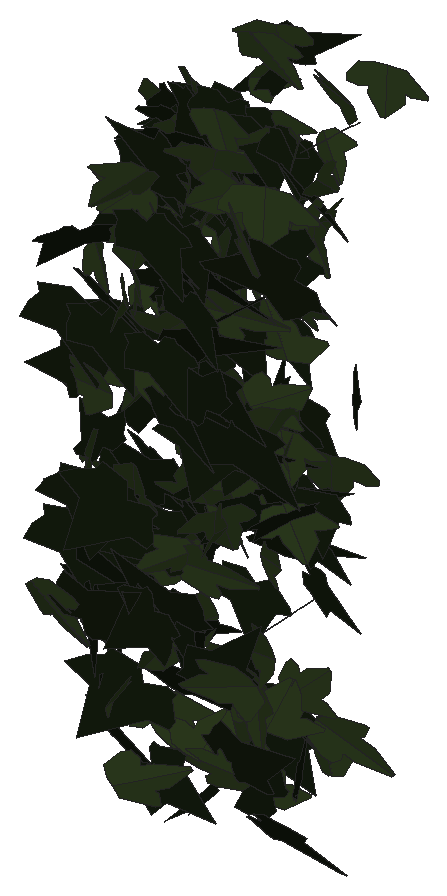
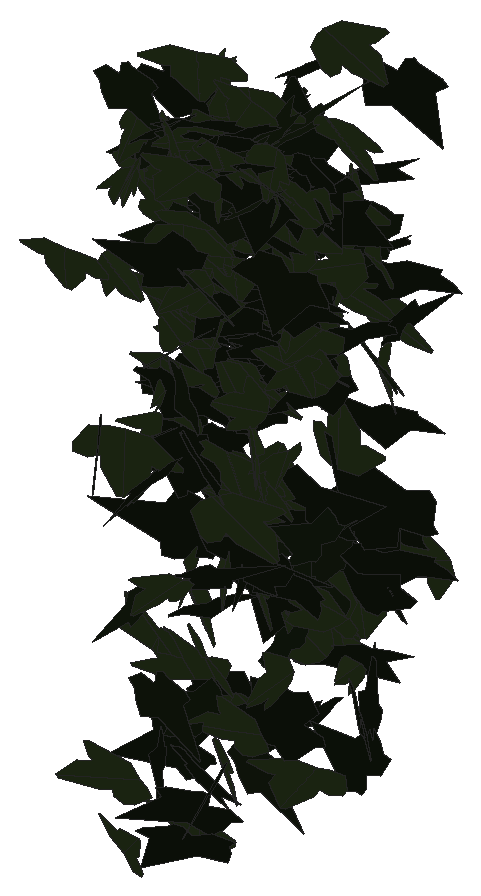
# SketchUp Ruby script. Lengths in millimetres.
U = 1.mm
M = Sketchup.active_model
def pt(a) = Geom::Point3d.new(a.map { |v| v * U })
def face(e, loops, mat)
  f = e.add_face(loops[0].map { |a| pt(a) })
  loops[1..].each { |l| e.add_face(l.map { |a| pt(a) }).erase! }
  f.material = f.back_material = mat if mat
  f
end
# faces: each face lists its corners as indices into pts; further lists are holes
def faces(e, pts, list, mat = nil) = list.each { |f| face(e, (f[0].is_a?(Array) ? f : [f]).map { |l| l.map { |i| pts[i] } }, mat) }
# xy, xz, yz: faces in a plane at the given z, y or x. An outline is a flat list of corners, or four numbers for a rectangle; further outlines are holes
def ring(l) = l.size == 4 ? [[l[0], l[1]], [l[2], l[1]], [l[2], l[3]], [l[0], l[3]]] : l.each_slice(2).to_a
def flat(e, list, mat, &to3) = list.each { |f| face(e, (f[0].is_a?(Array) ? f : [f]).map { |l| ring(l).map { |u, v| to3.(u, v) } }, mat) }
def xy(e, z, list, mat = nil) = flat(e, list, mat) { |x, y| [x, y, z] }
def xz(e, y, list, mat = nil) = flat(e, list, mat) { |x, z| [x, y, z] }
def yz(e, x, list, mat = nil) = flat(e, list, mat) { |y, z| [x, y, z] }
def lines(e, pts, list) = list.each { |a, b| e.add_line(pt(pts[a]), pt(pts[b])) }
# prism: a flat outline (further loops are holes) pulled along v
def prism(e, loops, v, mat = nil)
  f = face(e, loops, mat); d = Geom::Vector3d.new(v.map { |x| x * U })
  f.pushpull(f.normal.samedirection?(d) ? d.length : -d.length)
end
def box(e, o, s, mat = nil) = prism(e, [[o, [o[0] + s[0], o[1], o[2]], [o[0] + s[0], o[1] + s[1], o[2]], [o[0], o[1] + s[1], o[2]]]], [0, 0, s[2]], mat)
def at(x, y, z, deg = 0) = Geom::Transformation.translation(pt([x, y, z])) * Geom::Transformation.rotation(ORIGIN, Z_AXIS, deg.degrees)
def axes(o, x, y, z) = Geom::Transformation.new([*x, 0, *y, 0, *z, 0, *pt(o).to_a, 1])
def part(name) = M.definitions.add(name)
# library, detail: a bought-in or finely detailed component or shape, given as its bounding box
def library(name, o, s) = part(name).tap { |d| box(d.entities, o, s) }
def detail(e, o, s) = box(e.add_group.entities, o, s)
def put(e, d, t, mat = nil) = e.add_instance(d, t).tap { |i| i.material = mat if mat }
def group(e, t, mat = nil) = e.add_group.tap { |g| g.transformation = t; g.material = mat if mat }.entities
root = M.entities
M.materials.add("efeu1").color = [18, 25, 13]
M.materials.add("efeu2").color = [43, 57, 29]
c1 = part("ivyleaf_10")
p = [[0,12.8,-0.8],[-1.5,51.3,-10.9],[-4.9,51,-11.6],[-13.6,26.5,-7.3],[-13.2,15.9,-4.6],[-21.1,19.3,-7.2],
  [-29.5,16.3,-8.3],[-29.2,8.3,-6.2],[-19.7,-9.8,0.5],[-7.6,-13,4],[1,-12.2,5.8],[-0.4,51.1,-11.1],
  [-1.5,51.1,-10.9],[1,-12.4,5.9],[16.9,-12.4,3.5],[35.1,9.1,-5.1],[35,12.9,-6.1],[20.5,16.4,-4.9],
  [15.8,15,-3.8],[15.3,27.6,-7.1],[12.8,31.3,-7.8]]
faces(c1.entities,p,[[0,1,2,3,4,5,6,7,8,9,10],[11,12,0,13,14,15,16,17,18,19,20]],"efeu2")
c2 = part("ivyleaf_9")
p = [[39.1,54.8,31.7],[34.5,51.8,30.2],[-5.3,25.2,17.3],[-17.9,28.3,20.9],[-21.6,21.7,17],[-20.2,4.3,5.3],
  [-22.9,-0.3,2.5],[-17.1,-4,-0.6],[-2,-2.1,-1.2],[-0.7,-15.4,-10.1],[16.6,-22.3,-16.7],[21.1,-15.1,-12.5],
  [32.7,-10.7,-11],[46.1,-1.8,-6.6],[30.8,11.2,3.8]]
faces(c2.entities,p,[[0,1,2,3,4,5,6,7,8,9,10,11,12,13,14]],"efeu1")
put(root,c1,axes([4556.2,886.3,2542.8],[-1.01789,-0.02065,0.83927],[1.59777,-0.01294,0.53467],[-0.00035,0.99511,0.02437]))
put(root,c1,axes([4564.5,800.2,2431.5],[-0.15925,-0.13791,-1.07502],[1.36835,0.79977,-0.15856],[1.54355,-0.72322,0.02966]))
put(root,c2,axes([4578,723.1,2008.1],[-1.48385,-0.90702,-0.51552],[0.68416,0.37061,-1.19572],[1.86399,-0.85807,0.02849]))
put(root,c2,axes([4589.1,884.2,2448.3],[1.00623,0.8494,0.01435],[-0.12424,0.05747,-0.99682],[-1.61203,0.52577,0.08578]))
put(root,c1,axes([4580.1,1062.6,2511.9],[0.29812,0.25276,0.98298],[0.01179,0.99436,-0.25667],[-1.93162,0.04508,0.15014]))
put(root,c1,axes([4590.7,898.3,1915.5],[0.05878,0.11792,1.18277],[-0.48253,1.15659,-0.10869],[-2.21014,-0.24938,0.05519]))
put(root,c2,axes([4562.9,879.8,2561.1],[-0.31901,-0.00421,-0.99195],[1.88694,-0.03292,-0.16739],[-0.06044,-1.00548,0.00963]))
put(root,c1,axes([4594.7,1074.8,2581.2],[-1.55595,-0.56385,-0.01805],[0.12923,-0.0668,-0.98872],[1.06587,-0.81501,0.09352]))
put(root,c2,axes([4602.9,672.6,2277.1],[-0.44868,-0.18916,1.08119],[-1.24522,-0.86368,-0.29377],[1.67727,-0.69181,0.07113]))
put(root,c2,axes([4588.7,882.6,2406.1],[-1.19193,-0.69699,-0.34339],[0.4298,0.25873,-0.93701],[1.41492,-0.66573,-0.00464]))
put(root,c2,axes([4615.5,1063,2540],[-1.43483,0.68328,-0.16283],[0.23834,-0.10429,-1.01745],[-1.31542,-0.76421,-0.00674]))
put(root,c2,axes([4603.7,784.6,2473.6],[-0.07835,0.14297,-1.10614],[0.505,-1.07385,-0.14867],[-2.06176,-0.26846,0.00562]))
put(root,c1,axes([4571,734.4,2406.6],[0.64735,-0.2863,0.97578],[1.41515,-0.63187,-0.44459],[1.32025,0.81767,-0.00191]))
put(root,c2,axes([4577.1,786.8,2077.3],[0.3731,-1.04949,-0.00303],[0.00253,0.00333,-1.06764],[1.9974,0.19603,0.00192]))
put(root,c1,axes([4607.4,861.8,2487.1],[-1.5951,-0.65835,0.06001],[-0.07709,-0.04559,-1.06571],[1.2558,-0.83902,0.01081]))
put(root,c1,axes([4600.5,857.5,2305.2],[0.63665,0.81783,-0.44955],[-0.45449,-0.38665,-0.88109],[-1.71702,0.40559,0.06653]))
put(root,c2,axes([4586.6,758.1,1813],[-0.75692,0.17693,-1.07008],[1.82045,-0.4801,-0.43488],[-0.97314,-1.03574,0.01878]))
put(root,c2,axes([4617.2,822.9,2549.4],[0.46753,0.88942,-0.62998],[-0.37153,-0.59944,-0.92242],[-2.04081,0.31289,0.0236]))
put(root,c2,axes([4565.5,715.1,2049.6],[2.44799,0.26152,-0.16077],[0.2964,0.0409,1.31254],[0.50348,-1.29561,0.00898]))
put(root,c1,axes([4619.6,842.2,2526.7],[-1.77865,-0.22475,0.28094],[-0.52628,-0.05155,-0.9611],[0.43804,-0.97451,-0.01395]))
put(root,c2,axes([4596.3,724.5,1777.2],[0.27027,0.38621,1.16865],[-0.748,-1.10058,0.41147],[2.21984,-0.41788,-0.00364]))
put(root,c1,axes([4578.7,627.4,1960.3],[-1.14106,0.4755,-0.89578],[1.30933,-0.57389,-0.76508],[-1.41816,-0.91244,0.01439]))
put(root,c1,axes([4615.8,884,2593.4],[-1.44399,0.61214,0.2255],[-0.38212,0.10997,-0.97407],[-1.1813,-0.78384,0.03944]))
put(root,c2,axes([4581.2,837.7,2072.2],[0.73389,-0.86651,0.45505],[0.40083,-0.40417,-0.9481],[1.81907,0.43864,0.02533]))
put(root,c1,axes([4592.2,1047,2575.4],[-1.53117,0.15219,-0.61559],[1.07106,-0.28695,-0.80643],[-0.5562,-0.97153,0.14175]))
put(root,c2,axes([4592.3,802.4,2529.4],[0.55445,-0.97442,-0.31232],[-0.14144,0.30373,-1.01693],[1.94231,0.30027,0.0151]))
put(root,c2,axes([4600.4,754.5,2313.2],[-0.35988,-1.0455,-0.36243],[0.06215,0.36225,-1.06202],[2.10505,-0.18943,-0.03061]))
put(root,c2,axes([4647.8,774.1,2070],[0.13444,-0.08019,1.08996],[-1.54625,0.72671,0.10612],[-1.39127,-0.81541,-0.01261]))
put(root,c1,axes([4648.1,643,2274.6],[0.41932,-0.17233,-1.04982],[-1.60413,0.6259,-0.27963],[1.23547,0.87115,-0.00676]))
put(root,c2,axes([4587.8,1090.2,2547.4],[0.2442,0.07802,0.98269],[1.79038,0.28649,-0.14558],[-0.56074,0.94872,-0.03686]))
put(root,c2,axes([4646.6,884.6,2562.2],[-1.69221,0.45497,0.07745],[-0.31001,-0.15206,-0.97668],[-0.82184,-0.87946,0.20894]))
put(root,c2,axes([4607.4,676.5,2362.5],[-1.42898,-0.89142,-0.58993],[0.73571,0.44569,-1.16547],[1.89672,-0.84446,0.00762]))
put(root,c2,axes([4628.6,712.7,1939.7],[1.62408,-0.41988,0.80531],[-1.33457,0.39762,0.95037],[-1.09844,-1.10391,0.03601]))
put(root,c1,axes([4615.6,840.9,2560.2],[-0.80724,-0.71462,-0.56248],[0.56916,0.47653,-0.83094],[1.63458,-0.51885,0.01155]))
put(root,c2,axes([4602.5,681.1,1919.7],[-0.31423,0.70017,0.81678],[0.36351,-0.79414,0.71937],[2.01496,0.25246,-0.0024]))
put(root,c1,axes([4607.4,890.4,2541.2],[-0.35672,0.4667,-0.86016],[0.43813,-0.83019,-0.5006],[-1.81023,-0.2929,0.04834]))
put(root,c2,axes([4633.9,842,2564.4],[1.42432,0.43766,-0.76082],[-1.30135,-0.33618,-0.86598],[-1.04738,1.01287,0.04132]))
put(root,c2,axes([4626.8,881.9,2547.5],[1.37489,0.60815,-0.343],[-0.57756,-0.17102,-0.94235],[-1.19676,0.7812,0.06073]))
put(root,c2,axes([4591,742,1722.2],[0.56627,-0.59523,0.94998],[0.72797,-0.86999,-0.66491],[2.00556,0.48385,-0.02689]))
put(root,c1,axes([4605.5,773.7,2357.6],[-0.3705,0.12924,1.16872],[1.41357,-0.90487,0.22378],[1.7349,0.76487,0.06726]))
put(root,c1,axes([4621.5,853.6,2181.5],[0.37836,1.03837,-0.09617],[-0.03412,-0.09448,-1.05723],[-1.98439,0.19961,-0.00016]))
put(root,c2,axes([4654.3,887.4,2563.3],[-1.49063,-0.30522,0.54424],[-0.91345,-0.26347,-0.83846],[0.7589,-0.91664,0.05978]))
put(root,c1,axes([4610.7,809.9,2328.2],[1.34686,0.57922,0.41777],[0.54636,0.30781,-0.91306],[-1.24454,0.76197,0.05128]))
put(root,c2,axes([4603.1,776.3,2020.6],[1.29782,-0.83193,-0.06586],[-0.06782,0.05594,-1.07566],[1.58683,0.6828,0.00789]))
put(root,c2,axes([4607.9,853.6,2027.1],[-0.75545,-0.04592,-0.95874],[1.79522,0.17331,-0.39883],[0.33802,-1.02309,-0.02453]))
put(root,c1,axes([4618.8,770,1941.2],[-0.4051,-0.85941,0.88653],[0.39441,0.86198,0.88537],[-2.31657,0.29704,-0.00429]))
put(root,c1,axes([4640.8,690.1,1931.8],[-1.398,-0.94584,-0.00263],[0.01233,-0.0017,-1.19755],[1.80008,-0.73456,0.00616]))
put(root,c1,axes([4644,735.9,2456.3],[-1.48011,-0.98029,0.00301],[-0.0047,-0.00188,-1.25131],[1.8657,-0.7777,-0.00076]))
put(root,c2,axes([4641.7,746.4,1978.5],[-0.92891,0.83569,-0.60486],[-0.57751,0.52324,0.96778],[1.87652,0.57471,-0.00157]))
put(root,c2,axes([4653,883.9,2486],[-1.87523,-0.15087,-0.10176],[0.19409,0.00626,-0.99674],[0.28685,-0.99052,0.0092]))
put(root,c1,axes([4642.7,824.7,2492],[0.97671,-0.83155,-0.41195],[-0.17698,0.4223,-0.96828],[1.75727,0.50471,0.13145]))
put(root,c1,axes([4643.7,883.1,2209.5],[0.46467,-0.88004,-0.54564],[-0.07283,0.55255,-0.90831],[1.96935,0.22808,0.09515]))
put(root,c1,axes([4639.4,828.4,2337.9],[-0.11057,0.15609,-1.05329],[-0.29571,-1.04481,-0.14626],[-2.00483,0.1455,0.07966]))
put(root,c2,axes([4643.6,831.5,2376],[-1.50717,-0.69283,-0.12966],[0.19853,0.07767,-1.05216],[1.32671,-0.79869,0.01015]))
put(root,c2,axes([4620.5,898,2540.8],[0.38872,-0.97394,0.04392],[0.17164,-0.02581,-0.99167],[1.84754,0.20731,0.08288]))
put(root,c1,axes([4622.4,804.8,1736.4],[1.71872,0.704,0.37846],[0.55621,0.24066,-1.14501],[-1.41585,0.94913,0.00961]))
put(root,c2,axes([4666.5,631.6,2203.6],[-0.00273,0.58859,0.92022],[-0.43559,0.89963,-0.57578],[-2.03283,-0.19356,0.12214]))
put(root,c2,axes([4621.4,842,2510.5],[0.93662,-0.9195,-0.04882],[-0.04613,0.0424,-1.04291],[1.75185,0.49272,-0.00136]))
put(root,c1,axes([4672.5,898.5,2109.5],[-1.38994,-0.6283,0.73122],[-0.97862,-0.52211,-0.96219],[1.55207,-0.89188,0.04815]))
put(root,c2,axes([4629.5,657.7,1958.5],[-0.78913,0.22846,-1.176],[2.03014,-0.49602,-0.47246],[-1.03779,-1.14406,-0.03]))
put(root,c1,axes([4659.3,704.6,2539.5],[1.74526,-0.40513,-0.42947],[-0.76782,0.14927,-1.00222],[0.82041,1.00154,-0.02436]))
put(root,c2,axes([4615.5,680.1,2395.5],[1.31339,-0.88624,0.28676],[0.36521,-0.21397,-1.12307],[1.73477,0.71602,0.01933]))
put(root,c1,axes([4639.7,642.7,2193.7],[0.8029,-0.93876,0.71655],[0.82549,-0.58455,-1.0212],[2.09056,0.59136,0.12804]))
put(root,c1,axes([4659,668,1810.9],[0.32053,-0.09147,1.07306],[-0.62623,1.02979,0.13943],[-1.95164,-0.34546,0.1315]))
put(root,c1,axes([4648.4,876.3,2243.7],[0.039,-0.48905,0.90607],[0.03318,0.90628,0.48877],[-1.95931,0.00561,0.02631]))
put(root,c2,axes([4697.3,852.7,2012.4],[-0.61996,0.15785,1.01209],[-1.73629,0.43823,-0.36197],[-0.88648,-0.96871,0.00117]))
put(root,c1,axes([4664.7,735.8,2257.3],[-0.19852,-0.92547,0.56781],[-0.10262,-0.56531,-0.9313],[2.0639,-0.11713,0.00831]))
put(root,c2,axes([4648.3,729.7,2222],[0.24556,0.0871,-1.06262],[-0.53702,1.03499,0.05058],[1.95681,0.27311,0.14723]))
put(root,c2,axes([4674.3,696.9,1832.2],[-1.86106,-0.82422,0.26843],[-0.35591,-0.19454,-1.27858],[1.6109,-0.99519,0.02762]))
put(root,c2,axes([4656.3,838.5,2585.7],[-0.54014,-0.40205,0.91877],[-0.29207,-0.92619,-0.4527],[1.88621,-0.25855,0.193]))
put(root,c2,axes([4644.3,660.7,2364.2],[0.02371,-1.15684,-0.28258],[0.00991,0.28264,-1.15688],[2.2664,0.01086,0.00801]))
put(root,c2,axes([4679.5,566.3,2544.6],[0.0292,0.92396,-0.61627],[-0.03722,-0.61601,-0.92406],[-2.11342,0.02362,0.00776]))
put(root,c2,axes([4694.3,750,2023],[-1.45054,-0.34163,0.78875],[-1.3004,-0.39879,-0.83296],[0.99255,-1.02175,0.06139]))
put(root,c2,axes([4662.3,636.4,2134.3],[-1.58977,-0.7343,-0.38515],[0.54979,0.25473,-1.11218],[1.47922,-0.88386,-0.00056]))
put(root,c1,axes([4663.3,695.1,2100.6],[-2.08973,0.50083,0.28511],[0.48923,-0.12347,1.20682],[0.98166,1.12768,0.0055]))
put(root,c2,axes([4687.5,748.9,2553],[-0.1546,-1.19786,0.09461],[0.01665,0.09423,1.20061],[-2.2868,0.08167,0.00235]))
put(root,c1,axes([4702.1,670.6,2309.2],[1.31464,-0.00426,-0.99408],[-1.89141,0.02619,-0.69067],[0.04557,1.21023,0.01145]))
put(root,c2,axes([4661.3,877.2,2502],[-0.54604,-0.95809,-0.03676],[0.08165,0.0255,-0.99956],[1.82296,-0.28813,0.03376]))
put(root,c1,axes([4693.6,1081.5,2512.8],[0.65174,0.0888,-0.96523],[-1.05971,0.85597,-0.11879],[1.51004,0.56237,0.33323]))
put(root,c2,axes([4634.6,793.7,2348.6],[0.60695,0.01601,1.17296],[2.18172,0.25372,-0.31514],[-0.47383,1.18876,0.05146]))
put(root,c1,axes([4656.2,834.4,2119],[1.30433,-0.54383,0.62493],[0.93155,-0.38853,-0.8749],[1.27203,0.84218,-0.00008]))
put(root,c1,axes([4636.5,744.7,1927.3],[1.28334,-0.13921,1.01089],[1.86788,-0.24326,-0.68816],[0.53171,1.19055,-0.02241]))
put(root,c1,axes([4661.3,772.7,2302.6],[-1.66169,-0.50427,0.41981],[0.78495,0.12171,1.00395],[-0.97125,0.96111,0.09313]))
put(root,c1,axes([4641.3,774.1,2243.2],[-0.67587,-0.21894,0.97012],[1.73933,0.33446,0.41002],[-0.74655,0.97744,0.07701]))
put(root,c2,axes([4676.7,905,1758.3],[0.82926,-0.27691,-0.99762],[-1.27916,0.74764,-0.50107],[1.49881,0.79128,0.12432]))
put(root,c2,axes([4678.1,878.6,2504.6],[0.9628,0.77261,0.4094],[0.01509,0.46891,-0.89471],[-1.66404,0.45127,0.22877]))
put(root,c2,axes([4653.7,611.4,1958.9],[-0.68176,0.39749,1.00042],[1.25481,-0.75246,0.53505],[1.61956,0.75031,0.00658]))
put(root,c2,axes([4707.1,912.5,2014],[-0.72949,-0.83198,-0.45171],[-0.28659,-0.42754,0.91525],[-1.77881,0.41008,0.03779]))
put(root,c1,axes([4673.5,831.6,2440.9],[0.26119,-1.08276,-0.04315],[0.07078,-0.03876,1.09095],[-2.06113,-0.13854,0.03199]))
put(root,c1,axes([4675.5,727.5,1852.8],[-0.19155,-0.95278,0.44517],[0.0932,0.44247,0.95808],[-1.99933,0.11191,0.00201]))
put(root,c1,axes([4688.8,877.1,2510.9],[-0.10183,-1.00265,-0.12054],[0.0055,0.12056,-1.00407],[1.92198,-0.05347,-0.00351]))
put(root,c2,axes([4643.7,796.7,1792],[1.95928,-0.21255,0.50691],[0.94722,-0.09638,-1.05116],[0.44405,1.14345,0.00563]))
put(root,c1,axes([4686.3,888,2574.5],[1.74954,-0.36909,-0.14474],[-0.15841,0.17768,-0.9817],[0.73772,0.91347,0.13247]))
put(root,c2,axes([4681.2,865.7,2596.1],[-0.46877,-0.97162,-0.0316],[0.00999,0.03127,-1.00235],[1.85013,-0.24635,-0.0026]))
put(root,c2,axes([4700,810.1,2016.5],[0.28248,-0.06138,-1.12897],[-1.49666,0.81252,-0.14756],[1.54608,0.79776,0.06342]))
put(root,c1,axes([4684.9,866.6,2421.4],[1.78543,0.34984,-0.01559],[-0.06166,0.04231,-0.99993],[-0.66361,0.9373,0.05095]))
put(root,c2,axes([4697.3,879.3,2591.1],[-1.5061,-0.61537,-0.06535],[0.26032,-0.07047,-0.99273],[1.14862,-0.79091,0.1393]))
put(root,c1,axes([4698.4,629.8,2424.9],[0.27989,-0.7576,-0.84923],[0.00548,0.85653,-0.76361],[2.16591,0.09573,0.11168]))
put(root,c1,axes([4714.3,636.5,2607],[-0.74518,-0.8846,0.70552],[-0.57544,-0.63762,-0.96726],[2.07515,-0.49447,-0.01487]))
put(root,c2,axes([4679.4,872,2565.8],[-0.06708,-0.94211,0.37102],[0.14462,-0.37265,-0.93905],[1.92162,-0.00484,0.08362]))
put(root,c2,axes([4673.3,776.9,1874.2],[1.10693,-0.472,-0.92215],[1.33676,-0.59767,0.74892],[-1.4492,-0.91182,-0.01354]))
put(root,c1,axes([4712.4,846.4,2006.6],[-0.69792,0.6527,0.75917],[-0.86062,0.61334,-0.74575],[-1.7,-0.57846,0.06587]))
put(root,c1,axes([4716.7,731.1,2020.9],[-0.43375,-0.46669,0.92718],[-0.55397,-0.88245,-0.51572],[1.89628,-0.36454,0.06142]))
put(root,c2,axes([4720,886.8,2149.1],[0.02766,0.29885,1.02923],[-0.3354,1.01598,-0.29251],[-2.01196,-0.16526,0.06291]))
put(root,c1,axes([4713.1,776.4,2081],[-1.83316,-0.14803,-0.23744],[-0.43285,-0.08157,0.97348],[-0.31018,0.98867,0.04477]))
put(root,c2,axes([4729.4,787.5,2261.5],[-0.67917,-0.77533,-0.61729],[-0.42975,-0.57522,0.85303],[-1.83655,0.42132,0.02867]))
put(root,c1,axes([4709.8,849.1,2326.2],[0.28737,0.60151,-0.79965],[-0.064,0.81129,0.60392],[1.90332,-0.06354,0.14104]))
put(root,c1,axes([4672.9,856.7,1796.5],[0.73264,-0.06136,0.95296],[1.80203,0.15797,-0.37231],[-0.23603,1.01556,0.11549]))
put(root,c2,axes([4679.9,871.7,2534.4],[0.26585,-0.07753,-0.99855],[1.90194,-0.05626,0.14416],[-0.12676,-1.0067,0.06884]))
put(root,c2,axes([4716,865.5,2441.3],[-1.37012,-0.68236,-0.17883],[0.22403,0.13572,-0.99175],[1.32369,-0.72926,-0.01725]))
put(root,c1,axes([4730,816.5,2235.5],[1.14217,-0.50816,-0.7164],[-0.71665,0.63502,-0.76587],[1.51021,0.68566,0.17838]))
put(root,c1,axes([4719.3,870.2,2455.9],[1.8639,0.01814,-0.22956],[-0.43471,0.20366,-0.95838],[0.05556,0.98506,0.20237]))
put(root,c1,axes([4755,765.4,2199.1],[-0.2059,0.17491,1.03635],[-1.99499,0.05779,-0.11918],[-0.14543,-1.04038,0.16761]))
put(root,c2,axes([4687.8,918.9,1720.2],[0.31569,-0.30042,-0.96853],[0.73758,0.92568,-0.22076],[1.78343,-0.32966,0.26274]))
put(root,c1,axes([4720.3,738.3,2438.9],[-0.02629,-0.90295,0.70048],[0.23616,-0.69757,-0.89676],[2.16212,0.06522,0.10647]))
put(root,c1,axes([4700.5,815.7,2603.1],[1.66852,-0.21613,0.47187],[0.89176,-0.06876,-0.90204],[0.42481,0.99324,0.04023]))
put(root,c1,axes([4734.3,775.8,2581.1],[-1.75103,-0.59382,0.09037],[-0.1445,-0.04901,-1.09504],[1.13401,-0.92317,0.00001]))
put(root,c2,axes([4706.1,921.3,1673.9],[-0.457,-0.6266,-0.77616],[0.60449,0.70876,-0.67045],[1.79969,-0.39718,0.0281]))
put(root,c1,axes([4724.6,875.7,2531.3],[1.52018,0.62419,-0.04644],[-0.32504,0.14492,-0.98975],[-1.14604,0.78687,0.21912]))
put(root,c2,axes([4755.3,665.4,1969.8],[0.5431,-0.15616,1.05734],[-1.52326,0.69407,0.31852],[-1.34814,-0.84714,0.06606]))
put(root,c1,axes([4705.4,921.7,2556.7],[1.5935,0.21181,0.50987],[0.82483,0.32167,-0.84531],[-0.651,0.92602,0.17702]))
put(root,c2,axes([4728.1,720.8,1924.4],[1.15657,0.86851,-0.0681],[-0.08249,-0.05278,-1.05999],[-1.65598,0.60922,0.00524]))
put(root,c2,axes([4712.7,678.6,1735],[0.86789,-0.6841,-0.98124],[-0.67348,0.92597,-0.81002],[2.17466,0.55979,0.14075]))
put(root,c2,axes([4747.6,933.5,1864.8],[-0.60377,0.97874,-0.31163],[0.19188,-0.29491,-1.02886],[-1.94543,-0.33284,-0.00476]))
put(root,c1,axes([4743,753.7,1929.1],[0.67853,-0.67819,-0.65364],[-0.46742,0.60779,-0.76457],[1.73062,0.43006,0.04977]))
put(root,c1,axes([4722.2,1131.6,2536.9],[1.94061,0.0885,0.10843],[0.20708,0.00034,-1.02345],[-0.16756,1.02541,-0.00902]))
put(root,c1,axes([4746,814.8,1724.7],[0.49103,-0.77552,-0.70588],[-0.50583,0.65484,-0.81659],[1.93066,0.36881,-0.03442]))
put(root,c1,axes([4728.4,852.8,2400.3],[0.15878,0.99386,-0.10781],[-0.02473,-0.1071,-0.99735],[-1.90245,0.08434,0.00397]))
put(root,c2,axes([4756.5,747,1686.4],[-1.01304,0.9446,-0.37856],[0.34792,-0.33151,-1.08424],[-1.90525,-0.56279,0.00329]))
put(root,c2,axes([4694.2,758.7,2419.6],[1.5902,-0.52381,0.63201],[1.03259,-0.32434,-0.98609],[1.17236,0.99618,0.01127]))
put(root,c2,axes([4714.8,701.8,1970.5],[0.35199,-1.24807,0.37799],[0.09799,-0.37449,-1.26169],[2.47993,0.19194,-0.0038]))
put(root,c2,axes([4720.1,810.4,2324.5],[-0.82186,-0.50123,-0.85511],[1.02879,0.66273,-0.66145],[1.5812,-0.69173,-0.0141]))
put(root,c1,axes([4760.7,769.3,2541.1],[1.55459,-0.44863,-0.67769],[-1.11516,0.34076,-0.93183],[1.0719,1.00517,0.01343]))
put(root,c1,axes([4728,801.7,2441],[0.43713,-0.50762,0.92929],[0.90119,-0.80129,-0.55474],[1.80256,0.5237,0.05198]))
put(root,c2,axes([4739.1,642.1,1982],[0.53547,-0.59823,-1.15429],[0.96195,-1.03777,0.66104],[-2.27971,-0.57842,0.00781]))
put(root,c1,axes([4706.2,803.1,2335.9],[-0.10581,-0.14219,1.15468],[1.86933,0.61382,0.12288],[-1.18669,0.97959,0.09061]))
put(root,c1,axes([4730.8,926.3,2002.9],[0.56294,0.80071,0.57967],[0.43479,0.53331,-0.85325],[-1.83041,0.37294,-0.0244]))
put(root,c2,axes([4783.1,735.9,2218.7],[-0.24764,0.25225,1.18893],[-1.16187,1.02037,-0.2833],[-2.00017,-0.62395,0.01737]))
put(root,c1,axes([4742.9,794.3,2104],[2.37155,-0.24335,-0.01156],[-0.01476,0.02061,-1.26949],[0.46343,1.24597,0.01874]))
put(root,c1,axes([4736.7,745.8,1739.2],[1.76835,0.36434,-0.45422],[0.56623,0.43823,0.9601],[0.95263,-0.93679,0.27248]))
put(root,c2,axes([4744.2,840.9,1936.4],[-0.59406,-1.02487,0.06024],[-0.02123,-0.05958,-1.07133],[1.95379,-0.31227,0.00667]))
put(root,c1,axes([4749.4,853.9,1636.9],[2.15828,-0.11412,0.10794],[-0.20442,0.01072,1.13975],[-0.21816,-1.1391,-0.00008]))
put(root,c2,axes([4733,711.8,2501.4],[0.04769,-1.20715,0.33415],[0.1486,-0.33206,-1.20546],[2.37921,0.04493,0.06859]))
put(root,c1,axes([4738.8,841.4,2559],[-0.00017,0.02567,1.05537],[0.52641,1.0185,-0.02475],[-1.93898,0.27651,-0.00681]))
put(root,c1,axes([4792.3,741.6,1724.6],[0.25014,0.08378,0.99588],[-1.77233,-0.35433,0.15271],[0.69041,-0.93995,0.03119]))
put(root,c2,axes([4747.6,858.1,2583.1],[-0.78767,-0.8742,-0.30009],[0.40349,0.23025,-0.96312],[1.71217,-0.45643,0.08891]))
put(root,c1,axes([4767.6,839.5,1983.1],[-0.47253,0.62545,0.83654],[-0.69321,0.75403,-0.67186],[-1.86311,-0.43918,0.03781]))
put(root,c2,axes([4758.2,744,2198.6],[-1.06879,-1.07736,0.16593],[-0.11331,-0.15606,-1.21479],[2.07152,-0.5644,0.01916]))
put(root,c2,axes([4737.2,684.1,2463.8],[2.08369,-0.72481,-0.33774],[0.54484,-0.17939,1.31299],[-1.421,-1.13161,0.00818]))
put(root,c2,axes([4743,890.6,2302.1],[0.37697,-1.07852,-0.14883],[-0.05703,0.14582,-1.09655],[2.07131,0.2003,-0.0031]))
put(root,c2,axes([4747.9,930.7,2147.6],[0.67132,-0.84193,-0.60469],[-0.48806,0.54801,-0.91261],[1.9115,0.43561,-0.02065]))
put(root,c2,axes([4770,845.1,2202.4],[0.24124,0.21286,1.05108],[0.33265,1.04015,-0.23172],[-2.01374,0.19732,0.08764]))
put(root,c1,axes([4727.9,733.7,2004],[-0.33983,-0.08973,1.07178],[1.97413,0.27282,0.19565],[-0.54108,1.05174,0.04068]))
put(root,c1,axes([4780.8,951.2,1643],[1.36811,-0.43025,0.61389],[-1.00017,0.31731,0.83776],[-1.01745,-0.89045,0.00192]))
put(root,c2,axes([4753.8,616,2558.1],[0.08998,-1.1338,-0.26417],[0.08717,0.266,-1.13343],[2.21393,0.03561,0.05536]))
put(root,c2,axes([4809.1,792.9,1675.7],[-1.25366,0.19108,-0.76987],[-1.43593,0.15802,0.68477],[0.46608,1.00082,0.03887]))
put(root,c2,axes([4760.3,627.7,2378.7],[0.00562,-1.058,-0.30134],[-0.00177,0.30134,-1.058],[2.09366,0.00309,-0.00009]))
put(root,c1,axes([4781,871.4,2569.7],[0.86935,-0.8954,-0.18049],[0.00699,0.2036,-1.00075],[1.73839,0.44696,0.09429]))
put(root,c2,axes([4748.7,849.3,1786.8],[0.64221,-0.86068,0.59164],[0.64537,-0.49778,-0.91755],[1.88004,0.46488,0.11287]))
put(root,c2,axes([4746.2,731.2,2285.1],[-0.23796,-0.20114,-1.0869],[1.98232,0.34473,-0.18361],[0.70424,-1.03833,0.14959]))
put(root,c2,axes([4738.7,746.1,2172.4],[1.4491,0.17439,1.00684],[1.8635,0.23464,-0.78109],[-0.55627,1.24033,0.0062]))
put(root,c2,axes([4758.8,645.7,2293.7],[0.90559,-0.99644,-0.07122],[-0.05161,0.06597,-1.10421],[1.90056,0.47658,0.00395]))
put(root,c1,axes([4754.3,572.3,1775.9],[0.68276,0.20737,-1.07011],[1.69012,0.59767,0.41353],[1.20296,-0.9574,0.02636]))
put(root,c2,axes([4785.1,771.7,2185.2],[-0.82887,-0.89185,0.20402],[-0.17559,-0.18199,-0.9925],[1.73234,-0.44517,-0.00298]))
put(root,c1,axes([4783.3,943.6,2544.6],[0.13124,1.00786,-0.02215],[0.00679,-0.02245,-1.01021],[-1.91862,0.06886,-0.00509]))
put(root,c2,axes([4805.8,773.7,2101.2],[-0.03194,0.49688,-0.9755],[-0.01862,-0.97564,-0.49679],[-2.08346,0.0011,0.01939]))
put(root,c1,axes([4775.4,811.1,2517.9],[1.74946,0.45637,0.34547],[0.56125,0.18256,-1.02582],[-0.93366,0.96488,0.03068]))
put(root,c2,axes([4784.3,871.1,2570.8],[-0.22737,-1.01271,0.05879],[-0.04315,-0.05652,-1.01961],[1.93015,-0.12056,-0.01587]))
put(root,c2,axes([4765.9,660,2370.5],[1.19028,0.27606,1.02935],[1.76641,0.44551,-0.68339],[-0.99688,1.11903,0.01813]))
put(root,c1,axes([4820.7,769.3,1891.6],[0.53411,-0.54548,-1.0018],[-0.75665,0.9202,-0.61243],[2.03481,0.48536,0.03522]))
put(root,c1,axes([4808.5,820.4,2310.8],[1.96364,0.22803,0.28353],[-0.52658,-0.06193,1.05665],[0.4497,-1.06821,-0.00074]))
put(root,c2,axes([4816.5,953,2192.7],[0.37619,-0.11246,-1.01213],[-1.55552,0.59753,-0.22601],[1.15619,0.8405,0.02525]))
put(root,c2,axes([4761.1,833.8,2019.4],[1.04494,-0.15476,0.95297],[1.80435,-0.12076,-0.56582],[0.34725,1.09317,0.0724]))
put(root,c2,axes([4796.4,822.7,2198.5],[-1.30413,-0.28473,-0.77919],[1.36902,0.29953,-0.74203],[0.78653,-0.99346,-0.0004]))
put(root,c2,axes([4782.6,842.2,2415.9],[1.17439,-0.77703,0.18831],[0.26148,-0.13128,-0.99191],[1.49902,0.63166,0.0255]))
put(root,c2,axes([4832,710,2426.3],[-0.21875,1.19731,-0.10819],[0.01805,-0.10778,-1.20282],[-2.28794,-0.11533,0.00085]))
put(root,c2,axes([4799.9,889.9,1943.9],[1.26521,-0.6276,-0.5162],[-0.62648,0.40178,-0.91242],[1.414,0.73957,0.05763]))
put(root,c1,axes([4793.9,776.6,1813.9],[1.40499,-0.5197,0.78557],[1.1627,-0.49551,-0.9019],[1.36446,0.95737,-0.04036]))
put(root,c2,axes([4796.5,797.7,2097],[0.33465,0.68573,-0.90844],[0.05483,0.91624,0.69719],[2.16552,-0.12917,0.12274]))
put(root,c2,axes([4847.4,611.8,2330.6],[-0.12421,0.41749,1.02702],[-0.86636,0.92798,-0.40616],[-1.92389,-0.44484,0.1166]))
put(root,c2,axes([4825,826.2,1678.2],[0.03426,-0.22074,1.05801],[0.62627,1.00904,0.20492],[-1.95931,0.31867,0.084]))
put(root,c1,axes([4823.1,674.7,2136],[-1.1491,-0.98821,-0.40076],[0.41602,0.33607,-1.15801],[1.98645,-0.64203,0.01069]))
put(root,c2,axes([4793.1,739.1,1743],[-0.21742,0.14574,1.08683],[1.28508,-0.85163,0.18517],[1.64439,0.68481,-0.00101]))
put(root,c2,axes([4799.1,856.6,2539.6],[1.12999,-0.82559,0.0581],[0.05502,-0.05077,-1.0169],[1.57418,0.59441,-0.00616]))
put(root,c1,axes([4836.9,766,2245.9],[-0.93412,-1.09543,0.24458],[-0.16635,-0.22883,-1.20028],[2.12967,-0.49835,0.01352]))
put(root,c1,axes([4839.4,796.3,2176.3],[-0.0066,-0.06408,1.04411],[-0.75428,0.96636,0.05799],[-1.84248,-0.39538,-0.02748]))
put(root,c2,axes([4851.9,866.5,2611.9],[-0.59953,0.91287,-0.35343],[0.0502,-0.36323,-0.96169],[-1.86236,-0.30366,0.08786]))
put(root,c1,axes([4842.8,876.1,2131.5],[-2.2167,-0.38803,0.0493],[-0.08563,-0.02094,-1.22765],[0.7395,-1.16558,0.00564]))
put(root,c2,axes([4812.6,619.8,2468.8],[0.42054,-1.07032,0.18904],[0.06059,-0.18645,-1.09287],[2.06768,0.22316,-0.00642]))
put(root,c1,axes([4818.9,780.5,1794.4],[1.82057,0.53186,-0.42665],[0.71143,0.20567,1.0945],[1.08528,-1.02702,-0.00177]))
put(root,c1,axes([4804.8,785.5,2245.6],[1.42012,-0.33143,-0.64862],[1.26424,-0.0713,0.80062],[-0.56871,-0.9861,0.16011]))
put(root,c1,axes([4846.3,853.4,2488.9],[0.21265,0.42951,0.91597],[-0.79473,0.85895,-0.35183],[-1.75374,-0.33716,0.2705]))
put(root,c1,axes([4840.9,849.2,2551.1],[-0.37224,-0.71341,-0.80037],[0.34622,0.7797,-0.73944],[2.01096,-0.26629,-0.02085]))
put(root,c2,axes([4875,774.7,2486.4],[-1.83106,0.14444,0.342],[-0.64655,0.04059,-0.97283],[-0.28495,-1.02027,0.00972]))
put(root,c1,axes([4826.9,790.5,2196.2],[1.90998,0.14723,0.24905],[0.46179,0.06135,-1.014],[-0.29988,1.03218,0.02474]))
put(root,c2,axes([4806.9,715.9,2234.3],[-0.49576,-0.3477,-1.1571],[2.0067,0.51257,-0.39138],[1.12281,-1.06958,0.18859]))
put(root,c2,axes([4829.2,650.2,1918.8],[-0.54594,-0.30355,1.04085],[1.77357,0.48128,0.39718],[-1.05469,0.96645,0.12913]))
put(root,c1,axes([4863.9,682,2516.2],[-0.99863,1.0044,-0.57786],[-0.49506,0.51606,1.13317],[2.14908,0.5856,-0.00748]))
put(root,c1,axes([4808.6,915.9,1713.8],[0.98723,0.05072,1.0102],[1.84781,0.29336,-0.51327],[-0.53977,1.09705,0.09055]))
put(root,c1,axes([4853.6,623.6,2148.7],[-0.07526,-0.5253,-0.98037],[0.05455,0.98018,-0.52636],[2.1161,-0.04395,-0.0213]))
put(root,c1,axes([4842.2,845,2509.1],[0.33684,-0.79659,0.68255],[0.65813,-0.6092,-0.80066],[1.88489,0.35506,0.15759]))
put(root,c2,axes([4841.4,821.7,2060.5],[1.04589,-0.67759,-0.64036],[-0.68884,0.52997,-0.87139],[1.63519,0.65665,0.0425]))
put(root,c2,axes([4864.9,428.1,2281.6],[-1.32419,-0.9607,0.68415],[-0.67153,-0.5884,-1.18507],[2.14185,-0.77843,0.05142]))
put(root,c1,axes([4847.7,730.6,2576.7],[2.08495,0.54995,-0.00416],[-0.00758,-0.00134,-1.22579],[-1.04667,1.0955,0.00059]))
put(root,c1,axes([4832.5,833.8,2487.6],[1.12479,-0.3393,0.87922],[1.49068,-0.40029,-0.68097],[0.99743,0.98085,0.02624]))
put(root,c2,axes([4851.5,833.6,2109.9],[-0.23388,-1.06042,0.18662],[-0.03711,-0.18561,-1.06752],[2.04887,-0.12441,0.00197]))
put(root,c1,axes([4895.1,621.3,1939.9],[1.24046,-0.1511,-0.89316],[-1.64498,0.22558,-0.6689],[0.51599,1.08243,0.01472]))
put(root,c1,axes([4843.8,805.7,1833.6],[1.58931,-0.44126,-0.51034],[0.8575,-0.23968,0.94449],[-0.95569,-0.94887,-0.00125]))
put(root,c1,axes([4857.4,768.9,2105.9],[1.31713,0.83972,0.21674],[0.26803,0.16479,-1.08815],[-1.62862,0.70623,-0.0038]))
put(root,c1,axes([4846.6,790.3,2407.5],[-0.95963,-0.1011,0.93447],[1.68575,-0.40592,0.43402],[0.59854,0.98117,0.27584]))
put(root,c2,axes([4843.6,743.3,1668.7],[1.792,-0.2457,0.27985],[0.5141,-0.07318,-0.9731],[0.48789,0.97955,-0.0025]))
put(root,c2,axes([4894.4,718.1,2144.3],[-0.14082,1.01548,-0.36408],[0.05365,-0.36299,-1.01817],[-2.05241,-0.07916,-0.00164]))
put(root,c2,axes([4926,687.1,2509.7],[-0.32378,-0.01016,-1.25752],[-2.1985,-0.5003,0.16032],[-0.94598,1.16619,0.05782]))
